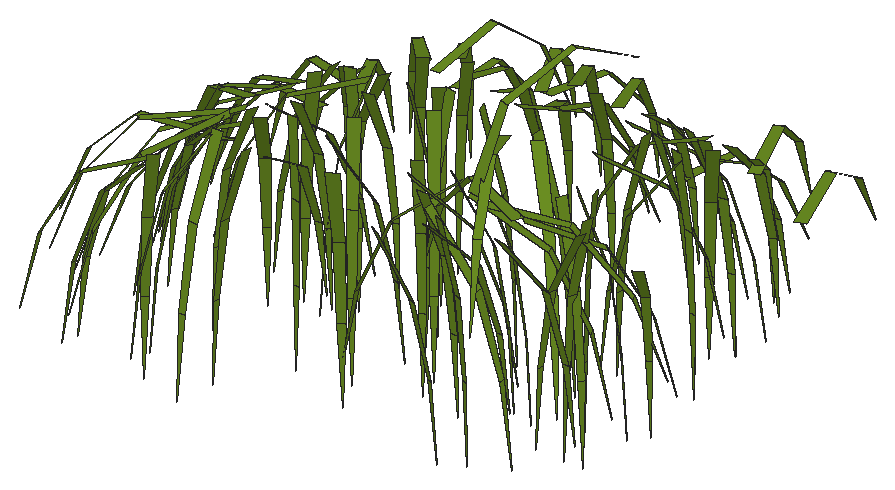
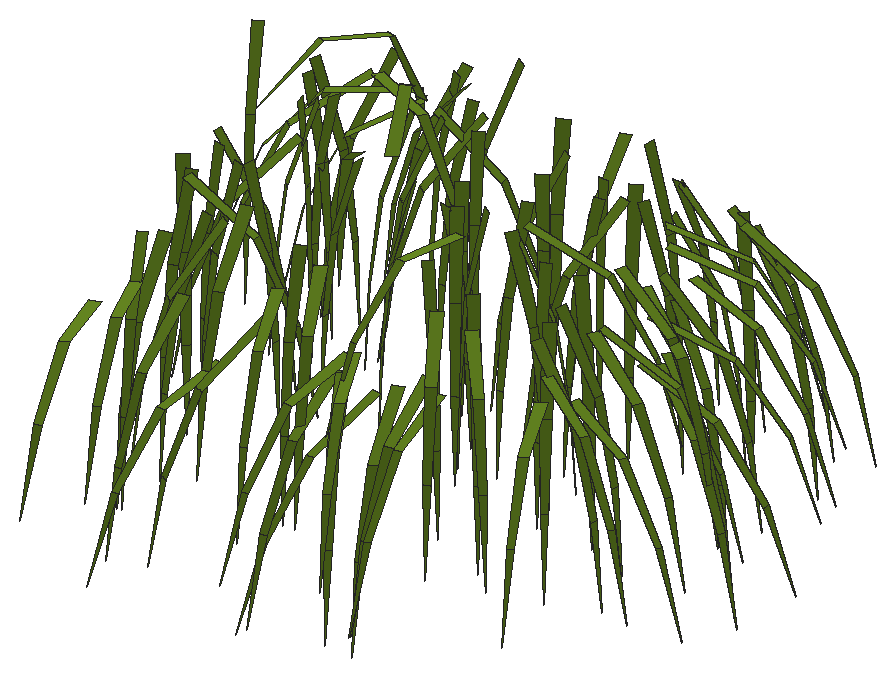
# SketchUp Ruby script. Lengths in inches.
U = 1.inch
M = Sketchup.active_model
def pt(a) = Geom::Point3d.new(a.map { |v| v * U })
def face(e, loops, mat)
  f = e.add_face(loops[0].map { |a| pt(a) })
  loops[1..].each { |l| e.add_face(l.map { |a| pt(a) }).erase! }
  f.material = f.back_material = mat if mat
  f
end
# faces: each face lists its corners as indices into pts; further lists are holes
def faces(e, pts, list, mat = nil) = list.each { |f| face(e, (f[0].is_a?(Array) ? f : [f]).map { |l| l.map { |i| pts[i] } }, mat) }
# xy, xz, yz: faces in a plane at the given z, y or x. An outline is a flat list of corners, or four numbers for a rectangle; further outlines are holes
def ring(l) = l.size == 4 ? [[l[0], l[1]], [l[2], l[1]], [l[2], l[3]], [l[0], l[3]]] : l.each_slice(2).to_a
def flat(e, list, mat, &to3) = list.each { |f| face(e, (f[0].is_a?(Array) ? f : [f]).map { |l| ring(l).map { |u, v| to3.(u, v) } }, mat) }
def xy(e, z, list, mat = nil) = flat(e, list, mat) { |x, y| [x, y, z] }
def xz(e, y, list, mat = nil) = flat(e, list, mat) { |x, z| [x, y, z] }
def yz(e, x, list, mat = nil) = flat(e, list, mat) { |y, z| [x, y, z] }
def lines(e, pts, list) = list.each { |a, b| e.add_line(pt(pts[a]), pt(pts[b])) }
# prism: a flat outline (further loops are holes) pulled along v
def prism(e, loops, v, mat = nil)
  f = face(e, loops, mat); d = Geom::Vector3d.new(v.map { |x| x * U })
  f.pushpull(f.normal.samedirection?(d) ? d.length : -d.length)
end
def box(e, o, s, mat = nil) = prism(e, [[o, [o[0] + s[0], o[1], o[2]], [o[0] + s[0], o[1] + s[1], o[2]], [o[0], o[1] + s[1], o[2]]]], [0, 0, s[2]], mat)
def at(x, y, z, deg = 0) = Geom::Transformation.translation(pt([x, y, z])) * Geom::Transformation.rotation(ORIGIN, Z_AXIS, deg.degrees)
def axes(o, x, y, z) = Geom::Transformation.new([*x, 0, *y, 0, *z, 0, *pt(o).to_a, 1])
def part(name) = M.definitions.add(name)
# library, detail: a bought-in or finely detailed component or shape, given as its bounding box
def library(name, o, s) = part(name).tap { |d| box(d.entities, o, s) }
def detail(e, o, s) = box(e.add_group.entities, o, s)
def put(e, d, t, mat = nil) = e.add_instance(d, t).tap { |i| i.material = mat if mat }
def group(e, t, mat = nil) = e.add_group.tap { |g| g.transformation = t; g.material = mat if mat }.entities
root = M.entities
M.materials.add("[0061_OliveDrab]").color = [107, 142, 35]
p = [[550.11,21.29,553.3],[550.25,21.43,553.3],[550.08,21.45,550.68],[549.24,29.09,553.35],[549.29,29.29,553.35],[548.93,29.29,550.75],
  [559.71,34.42,553.29],[559.91,34.35,553.29],[559.98,34.88,550.71],[553.87,34.64,553.24],[554.06,34.76,553.24],[553.6,35.27,550.71],
  [552.81,34.65,553.26],[553,34.73,553.26],[552.64,35.34,550.73],[547.85,25.41,553.35],[547.93,25.58,553.35],[547.51,25.69,550.77],
  [546.58,26.92,553.23],[546.6875,27.11,553.23],[545.84,27.47,550.77],[546.375,27.2,553.16],[546.48,27.39,553.16],[545.48,27.81,550.77],
  [550.45,29.67,553.38],[550.625,29.79,553.38],[550.4,29.93,550.76],[546.18,25.6,553.38],[546.16,25.82,553.38],[545.23,25.63,550.93],
  [551.1,26.88,553.56],[551.24,27.06,553.56],[551.07,27.04,550.93],[560.84,34.95,553.45],[561.03,34.98,553.45],[560.84,35.57,550.9],
  [555.43,35.47,553.27],[555.62,35.44,553.27],[555.68,36.49,550.86],[549.72,27.6,553.58],[549.75,27.81,553.58],[549.47,27.74,550.97],
  [552.66,27.23,553.71],[552.87,27.28,553.71],[552.75,27.3,551.09],[552.4375,30.0625,553.74],[552.58,30.19,553.74],[552.39,30.26,551.12],
  [562.04,31.48,553.76],[562.24,31.44,553.76],[562.17,31.6,551.14],[555.42,35.49,553.54],[555.625,35.52,553.54],[555.38,36.375,551.07],
  [548.125,21.26,553.77],[548.2,21.46,553.77],[547.77,21.5,551.18],[548.1,23.9,553.91],[548.09,24.12,553.91],[547.6875,23.99,551.3125],
  [561.91,33.37,553.93],[562.13,33.43,553.93],[561.92,33.78,551.33],[559.81,36.35,553.65],[560.01,36.36,553.65],[559.9,37.58,551.33],
  [550.32,21.65,554.01],[550.24,21.84,554.01],[550.11,21.67,551.39],[557.81,31.59,554.03],[557.99,31.69,554.03],[557.8125,31.82,551.41],
  [546.45,29.8,553.84],[546.52,29.98,553.84],[545.39,30.29,551.49],[554.02,29.83,554.14],[554.15,29.97,554.14],[553.97,30.01,551.52],
  [562.45,31.98,554.125],[562.64,31.86,554.125],[562.72,32.2,551.52],[561.72,33.55,554.1],[561.88,33.64,554.1],[561.55,34.03,551.53],
  [552.59,34.7,553.97],[552.8,34.74,553.97],[552.51,35.52,551.47],[552.69,19.91,554.24],[552.5,19.91,554.24],[552.59,19.71,551.62],
  [548.6,20.23,554.24],[548.57,20.43,554.24],[548.2,20.28,551.65],[553.9,23.06,554.21],[554.09,23.04,554.21],[553.99,23.0625,551.59],
  [562.7,24.45,554.26],[562.65,24.64,554.26],[562.65,24.54,551.64],[552.78,25.82,554.18],[552.66,25.99,554.18],[552.59,25.82,551.56],
  [547.35,26.06,554.17],[547.32,26.24,554.17],[546.69,26.04,551.63],[555.71,26.83,554.27],[555.875,26.72,554.27],[555.83,26.83,551.64],
  [563.1875,28.38,554.26],[563.4,28.34,554.26],[563.3,28.41,551.64],[560.79,21.68,554.32],[560.98,21.58,554.32],[560.92,21.69,551.7],
  [556.29,21.94,554.36],[556.5,22.03,554.36],[556.36,22.07,551.74],[551.07,23.2,554.28],[551.125,23.39,554.28],[550.9375,23.33,551.66],
  [555.78,23.36,554.29],[555.6,23.24,554.29],[555.73,23.24,551.67],[562.88,23.37,554.33],[562.91,23.57,554.33],[562.81,23.49,551.71],
  [557.64,23.74,554.33],[557.8125,23.84,554.33],[557.66,23.89,551.71],[557.48,24.76,554.36],[557.3125,24.63,554.36],[557.45,24.625,551.74],
  [556.35,25.86,554.29],[556.15,25.89,554.29],[556.23,25.76,551.66],[558.48,26.8,554.35],[558.55,26.6,554.35],[558.61,26.73,551.72],
  [561.01,27.99,554.27],[561.02,28.22,554.27],[560.92,28.11,551.65],[562.38,29.33,554.29],[562.57,29.28,554.29],[562.51,29.42,551.67],
  [562.67,30.65,554.31],[562.87,30.7,554.31],[562.72,30.89,551.69],[553.05,20.7,554.41],[553.07,20.9,554.41],[552.93,20.8125,551.79],
  [547,23.57,554.32],[546.92,23.77,554.32],[546.21,23.34,551.82],[563.44,23.56,554.4],[563.36,23.39,554.4],[563.49,23.4375,551.77],
  [560.82,24.3125,554.42],[560.97,24.2,554.42],[560.97,24.36,551.79],[563.29,25.32,554.41],[563.45,25.16,554.41],[563.46,25.33,551.79],
  [560.77,26.42,554.39],[560.77,26.2,554.39],[560.9,26.3125,551.77],[562.48,29.92,554.45],[562.65,30.07,554.45],[562.43,30.14,551.83],
  [550.68,20.46,554.49],[550.6,20.64,554.49],[550.43,20.44,551.87],[560.26,20.83,554.53],[560.46,20.72,554.53],[560.47,20.98,551.91],
  [559.15,23.21,554.49],[559.35,23.22,554.49],[559.25,23.38,551.87],[560.18,24.375,554.54],[560.33,24.26,554.54],[560.34,24.43,551.92],
  [552.99,25.53,554.54],[553.18,25.57,554.54],[553.03,25.78,551.93],[552.37,27.28,554.55],[552.46,27.47,554.55],[552.17,27.5,551.94],
  [555.09,27.68,554.48],[555.27,27.81,554.48],[555.08,27.88,551.86],[552.16,35.13,554.3125],[552.34,35.17,554.3125],[552.01,36.23,551.93],
  [562.32,22.95,554.64],[562.37,23.14,554.64],[562.14,23.1,552.02],[554.26,26.83,554.57],[554.44,26.875,554.57],[554.3,27.05,551.96],
  [548.89,33.08,554.34],[549.07,33.18,554.34],[548.38,34.23,552.04],[547.33,20.33,554.66],[547.3125,20.55,554.66],[546.67,20.4,552.11],
  [556.375,24.27,554.71],[556.56,24.17,554.71],[556.59,24.44,552.1],[551.87,24.3,554.72],[552.05,24.42,554.72],[551.77,24.63,552.11],
  [547.21,28.46,554.54],[547.29,28.66,554.54],[546.39,28.91,552.09],[547.35,30.72,554.47],[547.44,30.89,554.47],[546.47,31.29,552.07],
  [562.96,23.25,554.89],[563.18,23.21,554.89],[563.13,23.54,552.28],[561.41,27.05,554.87],[561.4,27.24,554.87],[561.125,27.13,552.26],
  [562.43,21.38,555.01],[562.43,21.2,555.01],[562.78,21.29,552.4],[555.87,35.75,554.78],[556.08,35.74,554.78],[555.99,36.79,552.37],
  [560.8125,23.1,555.15],[561.02,23.07,555.15],[560.96,23.46,552.55],[559.89,24.53,555.1],[560.06,24.42,555.1],[560.18,24.8,552.51],
  [547.37,26.64,555.03],[547.46,26.83,555.03],[546.72,27.08,552.52],[564.9375,24.3,555.21],[565.09,24.4,555.21],[564.8,24.69,552.62],
  [559.88,32.47,555.15],[560.09,32.53,555.15],[559.84,32.97,552.57],[562.52,36.23,554.75],[562.72,36.3,554.75],[562.09,37.7,552.62],
  [547.93,26.11,555.28],[547.99,26.3125,555.28],[547.3,26.4,552.74],[553.48,26.33,555.3125],[553.68,26.29,555.3125],[553.67,26.82,552.74],
  [551.89,32.88,555.18],[552.07,33.01,555.18],[551.5625,33.55,552.66],[549.2,20.37,555.32],[549.06,20.53,555.32],[548.66,20.02,552.78],
  [556.78,22.08,555.42],[556.74,22.28,555.42],[556.29,22.09,552.84],[550.25,32.55,555.29],[550.4,32.68,555.29],[549.66,33.34,552.86],
  [556.77,34.63,555.39],[556.9375,34.72,555.39],[556.44,35.5,552.93],[546.26,23.77,555.38],[546.29,23.96,555.38],[545.13,24.04,553.02],
  [563.03,29.2,555.6],[563.23,29.11,555.6],[563.36,29.61,553.03],[553.4,35.27,555.4],[553.58,35.37,555.4],[552.86,36.43,553.11],
  [562.49,23.64,555.72],[562.33,23.48,555.72],[562.85,23.13,553.17],[563.4,23.97,555.72],[563.49,23.77,555.72],[563.95,24.09,553.15],
  [553.9375,23.94,555.77],[554.13,24,555.77],[553.87,24.53,553.21],[547.92,26.1,555.33],[548.07,26.36,555.33],[547.84,26.37,555.17],
  [547.99,26.64,555.17],[554.55,33.48,555.5],[554.82,33.65,555.5],[555.74,33.52,555.67],[555.93,33.64,555.67],[555.4375,34.25,553.17],
  [550.36,21.02,555.9],[550.54,21.23,555.9],[547.46,21.98,555.77],[547.4,22.17,555.77],[546.58,21.8,553.3],[559.3125,33.39,555.67],
  [559.6,33.29,555.67],[553.29,33.37,555.5],[553.5625,33.48,555.5],[555.14,33.82,555.29],[555.4,33.78,555.29],[560.98,35.61,555.58],
  [561.18,35.7,555.58],[560.5625,36.82,553.29],[548.6875,24.93,555.79],[548.81,25.16,555.79],[547.77,25.7,555.47],[547.74,26,555.47],
  [550.02,28.8125,555.84],[550.1,29.1,555.84],[550.78,29.125,555.93],[551.02,29.3,555.93],[559.27,29.27,555.9],[559.27,29.47,555.9],
  [558.5625,29.38,553.38],[560.99,33.7,555.75],[561.27,33.74,555.75],[550.53,24.83,556.05],[550.47,25.05,556.05],[549.83,24.76,553.52],
  [564.41,25.28,556.01],[564.59,25.15,556.01],[564.875,25.72,553.46],[555.64,33.9375,555.65],[555.92,33.98,555.65],[551.32,26.65,556.16],
  [551.52,26.9,556.16],[550.34,27.47,556.13],[550.38,27.77,556.13],[552.66,27.07,556.33],[552.95,27.14,556.33],[552.74,29.67,556.32],
  [552.94,29.85,556.32],[559.79,34.38,555.38],[560.06,34.38,555.38],[548.98,20.9,556.23],[549.08,21.17,556.23],[548.2,29.11,555.67],
  [548.29,29.36,555.67],[561.93,31.08,556.35],[562.21,31.03,556.35],[549.02,23.89,556.36],[549.01,24.21,556.36],[562.09,32.49,556.39],
  [562.4,32.57,556.39],[550.79,21.8,556.59],[550.68,22.07,556.59],[558.01,31.08,556.59],[558.27,31.21,556.59],[552.89,33.2,556.1],
  [553.1875,33.26,556.1],[554.33,29.49,556.72],[554.51,29.68,556.72],[562,31.39,556.64],[562.27,31.21,556.64],[562.23,32.58,556.49],
  [562.46,32.71,556.49],[552.74,20.36,556.82],[552.47,20.37,556.82],[549.49,20.3,556.71],[549.45,20.59,556.71],[553.85,23.03,556.84],
  [554.125,23,556.84],[553.12,26,556.77],[552.96,26.24,556.77],[548.64,26.24,556.45],[548.6,26.5,556.45],[560.66,21.51,556.94],
  [560.9375,21.38,556.94],[551.49,23.04,556.86],[551.5625,23.32,556.86],[555.72,23.53,556.91],[555.47,23.36,556.91],[563.1,23.29,556.95],
  [563.15,23.58,556.95],[557.73,23.49,556.94],[557.98,23.625,556.94],[548.4,24.13,556.47],[548.27,24.41,556.47],[562.79,24.43,556.88],
  [562.71,24.7,556.88],[556.42,26.11,556.9],[556.14,26.15,556.9],[555.57,26.69,556.88],[555.8,26.53,556.88],[558.23,26.76,556.96],
  [558.32,26.47,556.96],[561.27,27.9375,556.89],[561.28,28.25,556.89],[563.12,28.25,556.88],[563.41,28.19,556.88],[562.26,29.03,556.89],
  [562.53,28.96,556.89],[562.74,30.14,556.88],[563.02,30.2,556.88],[549.8,31.3,556.05],[550.0625,31.44,556.05],[552.53,33.31,556.17],
  [552.78,33.37,556.17],[553.37,20.61,557.01],[553.41,20.9,557.01],[556.35,21.6875,556.98],[556.65,21.82,556.98],[563.18,23.71,557],
  [563.08,23.47,557],[560.59,24.07,557.02],[560.8,23.91,557.02],[557.35,24.99,556.98],[557.12,24.8,556.98],[563.02,25.13,557.02],
  [563.24,24.9,557.02],[560.45,26.46,557],[560.46,26.14,557],[562.79,29.52,557.02],[563.02,29.73,557.02],[559.98,20.4,557.1],
  [560.25,20.25,557.1],[551.25,20.68,557.04],[551.13,20.93,557.04],[559.13,22.8,557.08],[559.41,22.81,557.08],[559.91,24.07,557.14],
  [560.125,23.91,557.14],[553.08,24.97,557.11],[553.34,25.03,557.11],[555.32,27.3,557.07],[555.5625,27.48,557.07],[548.68,27.83,556.62],
  [548.8,28.11,556.62],[548.92,29.85,556.4],[549.04,30.09,556.4],[562.82,22.78,557.21],[562.89,23.04,557.21],[554.34,26.33,557.15],
  [554.6,26.39,557.15],[552.92,26.96,557.1],[553.05,27.23,557.1],[548.64,20.38,556.93],[548.62,20.68,556.93],[556.06,23.76,557.27],
  [556.32,23.625,557.27],[552.24,23.67,557.24],[552.49,23.84,557.24],[564.71,24.13,557.18],[564.79,23.95,557.18],[565.23,24.21,555.85],
  [565.59,24.42,554.72],[563.26,34.11,556.11],[563.54,34.21,556.11],[555.8,33.9375,556.68],[556.09,33.93,556.68],[562.78,22.55,557.41],
  [563.08,22.49,557.41],[562.1,27.05,557.4],[562.08,27.32,557.4],[561.63,21.42,557.51],[561.63,21.16,557.51],[548.68,25.93,557.1875],
  [548.82,26.21,557.1875],[560.67,22.25,557.63],[560.97,22.21,557.63],[559.38,23.83,557.58],[559.63,23.67,557.58],[560.15,31.42,557.54],
  [560.45,31.51,557.54],[565.39,23.52,557.67],[565.61,23.66,557.67],[549.93,25.21,556.26],[550.11,25.54,556.26],[552.67,31.67,557.375],
  [552.93,31.85,557.375],[550.19,21.21,557.6],[549.99,21.4375,557.6],[558.08,23.97,557.69],[558.17,24.15,557.69],[557.19,24.48,555.27],
  [549.97,24.89,556.44],[550.15,25.2,556.44],[553.23,25.26,557.7],[553.52,25.21,557.7],[549.25,25.68,557.51],[549.33,25.97,557.51],
  [551.38,31.26,557.28],[551.59,31.46,557.28],[554.74,31.45,556.35],[555.06,31.4,556.35],[557.8,22.25,557.83],[557.74,22.53,557.83],
  [548.12,23.45,557.21],[548.16,23.71,557.21],[559.78,31.77,555.64],[560.12,31.77,555.64],[557.48,33.09,557.39],[557.72,33.21,557.39],
  [554.37,33.47,557.05],[554.62,33.62,557.05],[550.16,25.875,556.54],[550.125,26.25,556.54],[554.15,31.17,556.65],[554.49,31.3125,556.65],
  [555.78,31.46,556.64],[556.11,31.67,556.64],[562.5,28.24,557.99],[562.78,28.11,557.99],[561.78,33.71,557.2],[562.0625,33.83,557.2],
  [562.32,23.55,558.07],[562.44,23.27,558.07],[561.64,24.52,558.05],[561.43,24.3,558.05],[550.6,28.19,556.21],[550.71,28.5,556.21],
  [558.59,31.39,557.2],[558.9375,31.27,557.2],[556,31.54,556.65],[556.35,31.59,556.65],[555.09,32.09,558.04],[555.28,32.09,558.04],
  [555.24,32.5625,557.11],[555.17,33.28,555.7],[556.47,32.2,557.82],[556.74,32.35,557.82],[549.03,22.44,557.82],[548.94,22.72,557.82],
  [554.23,22.78,558.11],[554.5,22.86,558.11],[550.46,23.98,557.49],[550.6,24.26,557.49],[551.78,28.26,557.71],[551.88,28.61,557.71],
  [561.3125,31.42,557.02],[561.65,31.48,557.02],[551.05,20.37,558.35],[551.28,20.63,558.35],[551.67,27.8,558.01],[551.97,28.02,558.01],
  [560.67,29.2,558.12],[560.68,29.48,558.12],[564.15,31.64,555.95],[564.49,31.77,555.95],[563.61,24.27,558.29],[563.86,24.08,558.29],
  [551.02,28.99,556.31],[551.33,29.16,556.31],[551.875,25.15,558.28],[551.79,25.46,558.28],[551.8,27.24,558.3],[551.85,27.61,558.3],
  [553.41,30.8,557.03],[553.77,30.88,557.03],[550.8,20.18,557.98],[550.92,20.52,557.98],[551.93,26.13,558.66],[552.17,26.43,558.66],
  [553.0625,30.78,556.59],[553.37,30.85,556.59],[552.73,26.65,558.92],[553.08,26.73,558.92],[553.6,28.66,558.58],[553.85,28.88,558.58],
  [550.97,23.95,558.125],[550.95,24.33,558.125],[550.96,26.61,557.625],[550.91,26.92,557.625],[551.17,28.625,556.98],[551.32,28.92,556.98],
  [561.71,29.97,558.72],[562.05,29.91,558.72],[562.53,30.62,558.18],[562.91,30.72,558.18],[550.62,25.0625,557.51],[550.47,25.41,557.51],
  [563.29,30.71,558],[563.5625,30.87,558],[552.01,22.28,558.87],[551.87,22.6,558.87],[550.92,26.89,557.625],[551.0625,27.24,557.625],
  [558.62,29.77,558.79],[558.94,29.93,558.79],[561.09,30.0625,558.72],[561.42,29.85,558.72],[561.58,21.49,558.96],[561.39,21.375,558.96],
  [562.17,20.25,556.72],[551.4,20.52,558.49],[551.36,20.875,558.49],[555.21,28.6,559.03],[555.43,28.84,559.03],[555.73,31.35,557.11],
  [556.09,31.34,557.11],[552.78,21.42,559.22],[552.45,21.42,559.22],[553.8125,22.93,559.46],[554.15,22.9,559.46],[553.93,26.5,559.22],
  [553.73,26.8,559.22],[550.97,20.5,558.13],[550.95,20.87,558.13],[560.39,21.01,559.5],[560.73,20.85,559.5],[552.59,22.72,559.23],
  [552.68,23.06,559.23],[557.99,22.96,559.5],[558.29,23.13,559.5],[563.69,23.17,559.5],[563.75,23.52,559.5],[555.52,23.91,559.5],
  [555.21,23.71,559.5],[563,24.46,559.5],[562.9,24.79,559.5],[555.22,26.23,559.44],[555.52,26.04,559.44],[556.53,26.65,559.46],
  [556.18,26.7,559.46],[563.01,27.84,559.47],[563.37,27.77,559.47],[561.95,27.875,559.42],[561.97,28.26,559.42],[562.02,28.26,559.39],
  [562.36,28.17,559.39],[562.97,28.99,559.23],[563.32,29.07,559.23],[554.1875,20.47,559.5],[554.23,20.82,559.5],[552.6,21.29,559.21],
  [552.45,21.6,559.21],[556.61,21.02,559.5],[556.97,21.18,559.5],[560.05,23.41,559.5],[560.31,23.21,559.5],[562.45,24.06,559.5],
  [562.32,23.76,559.5],[562.39,24.57,559.5],[562.66,24.29,559.5],[556.93,25.57,559.5],[556.64,25.34,559.5],[559.66,26.47,559.5],
  [559.67,26.09,559.5],[557.6,26.57,559.5],[557.72,26.23,559.5],[563.63,28.53,559.3],[563.91,28.78,559.3],[559.43,19.48,559.5],
  [559.77,19.3,559.5],[559.14,21.79,559.5],[559.48,21.8,559.5],[559.2,23.17,559.5],[559.47,22.98,559.5],[553.34,23.65,559.36],
  [553.67,23.72,559.36],[554.61,25.1,559.45],[554.93,25.18,559.45],[554.2,26.29,559.29],[554.36,26.62,559.29],[555.9375,26.41,559.46],
  [556.23,26.64,559.46],[555.64,31.18,557.18],[555.94,31.35,557.18],[562.82,31.3,557.13],[563.16,31.45,557.13],[553.08,22.36,559.35],
  [553.39,22.57,559.35],[564.05,22.42,559.5],[564.14,22.74,559.5],[550.66,23.03,557.71],[550.71,23.35,557.71],[563.12,23.46,559.16],
  [563.23,23.21,559.16],[550.86,24.79,558.09],[551.04,25.13,558.09],[555.38,22.57,559.5],[555.7,22.4,559.5],[553.07,29.38,557.99],
  [553.33,29.62,557.99],[562.43,21.01,559.5],[562.8,20.93,559.5],[563.68,27.11,559.5],[563.66,27.43,559.5],[554.04,29.64,558.32],
  [554.36,29.86,558.32],[558.59,30.77,557.92],[558.89,30.92,557.92],[559.93,21.45,559.5],[559.93,21.13,559.5],[551.56,24.98,558.54],
  [551.66,25.33,558.54],[560.74,29.37,559.07],[561.11,29.48,559.07],[560.42,20.43,559.5],[560.79,20.38,559.5],[551.95,22.76,558.79],
  [551.69,23.04,558.79],[558.38,22.35,559.5],[558.6875,22.15,559.5],[566.38,21.91,559.5],[566.65,22.09,559.5],[552.82,23.21,559.29],
  [553.17,23.15,559.29],[559.78,23.17,559.52],[559.9,23.43,559.52],[559.79,22.63,559.5],[559.72,22.98,559.5],[551.45,23.19,558.51],
  [551.34,23.53,558.51],[557.71,30.02,558.61],[558.04,30.22,558.61],[560.1,26.0625,559.5],[559.83,25.79,559.5],[561.51,26.34,559.5],
  [561.85,26.17,559.5],[555.08,30.03,559.66],[555.34,30.03,559.66],[554.8125,20.63,559.5],[555.14,20.73,559.5],[560.28,22.72,559.5],
  [560.34,22.58,559.5],[560.43,22.37,559.5],[563.08,29.12,559.16],[563.09,29.47,559.16],[562.2,22.41,559.5],[562.29,22.35,559.5],
  [562.51,22.18,559.5],[554.21,25.75,559.32],[554.11,26.125,559.32],[560.49,23.45,560.3125],[560.22,23.3,560.3125],[560.93,22.14,559.49],
  [560.73,22.43,559.5],[560.875,22.11,559.5],[555.08,27.43,559.29],[555.4,27.43,559.29],[562.16,22.08,559.5],[562.31,22.4,559.5],
  [560.28,22.59,559.5],[560.65,22.53,559.5],[560.79,23.62,561.88],[560.49,23.67,561.88],[559.26,25.63,559.5],[558.93,25.4375,559.5],
  [560.93,26.14,562.65],[561.14,26.1,562.65],[561.41,28.43,561.45]]
faces(root,p,[[0,1,2],[3,4,5],[6,7,8],[9,10,11],[12,13,14],[15,16,17],[18,19,20],[21,22,23],
  [24,25,26],[27,28,29],[30,31,32],[33,34,35],[36,37,38],[39,40,41],[42,43,44],[45,46,47],
  [48,49,50],[51,52,53],[54,55,56],[57,58,59],[60,61,62],[63,64,65],[66,67,68],[69,70,71],
  [72,73,74],[75,76,77],[78,79,80],[81,82,83],[84,85,86],[87,88,89],[90,91,92],[93,94,95],
  [96,97,98],[99,100,101],[102,103,104],[105,106,107],[108,109,110],[111,112,113],[114,115,116],[117,118,119],
  [120,121,122],[123,124,125],[126,127,128],[129,130,131],[132,133,134],[135,136,137],[138,139,140],[141,142,143],
  [144,145,146],[147,148,149],[150,151,152],[153,154,155],[156,157,158],[159,160,161],[162,163,164],[165,166,167],
  [168,169,170],[171,172,173],[174,175,176],[177,178,179],[180,181,182],[183,184,185],[186,187,188],[189,190,191],
  [192,193,194],[195,196,197],[198,199,200],[201,202,203],[204,205,206],[207,208,209],[210,211,212],[213,214,215],
  [216,217,218],[219,220,221],[222,223,224],[225,226,227],[228,229,230],[231,232,233],[234,235,236],[237,238,239],
  [240,241,242],[243,244,245],[246,247,248],[249,250,251],[252,253,254],[255,256,257],[258,259,260],[261,262,263],
  [264,265,266],[267,268,269],[270,271,272],[273,274,275],[276,277,278],[279,280,281],[282,283,284],[285,286,19,18],
  [287,288,22,21],[289,290,10,9],[291,292,293],[294,295,1,0],[296,297,298],[299,300,7,6],[301,302,13,12],[303,304,37,36],
  [305,306,307],[308,309,16,15],[310,311,28,27],[312,313,4,3],[314,315,25,24],[316,317,318],[319,320,34,33],[321,322,323],
  [324,325,326],[327,328,52,51],[329,330,31,30],[331,332,40,39],[333,334,43,42],[335,336,46,45],[337,338,64,63],[339,340,55,54],
  [341,342,73,72],[343,344,49,48],[345,346,58,57],[347,348,61,60],[349,350,67,66],[351,352,70,69],[353,354,85,84],[355,356,76,75],
  [357,358,79,78],[359,360,82,81],[361,362,88,87],[363,364,91,90],[365,366,94,93],[367,368,100,99],[369,370,103,102],[371,372,112,111],
  [373,374,118,117],[375,376,121,120],[377,378,124,123],[379,380,127,126],[381,382,151,150],[383,384,97,96],[385,386,133,132],[387,388,106,105],
  [389,390,136,135],[391,392,139,138],[393,394,109,108],[395,396,142,141],[397,398,145,144],[399,400,199,198],[401,402,190,189],[403,404,148,147],
  [405,406,115,114],[407,408,154,153],[409,410,157,156],[411,412,130,129],[413,414,160,159],[415,416,163,162],[417,418,166,165],[419,420,172,171],
  [421,422,169,168],[423,424,175,174],[425,426,178,177],[427,428,181,180],[429,430,187,186],[431,432,211,210],[433,434,214,213],[435,436,193,192],
  [437,438,196,195],[439,440,184,183],[441,442,202,201],[443,444,205,204],[445,446,208,207],[447,448,449,450],[451,452,244,243],[453,454,226,225],
  [455,456,217,216],[457,458,220,219],[459,460,223,222],[461,462,235,234],[463,464,229,228],[465,466,232,231],[467,468,241,240],[469,470,449,238,237],
  [471,472,288,287],[473,474,253,252],[475,476,256,255],[477,478,479],[480,481,286,285],[482,483,250,249],[484,485,247,246],[486,487,262,261],
  [488,489,304,303],[490,491,259,258],[492,493,268,267],[494,495,338,337],[496,497,265,264],[498,499,274,273],[500,501,311,310],[502,503,302,301],
  [504,505,290,289],[506,507,271,270],[508,509,306,305],[510,511,280,279],[512,513,277,276],[514,515,342,341],[516,517,300,299],[518,519,328,327],
  [520,521,522,523],[524,525,292,291],[526,527,297,296],[528,529,283,282],[530,531,309,308],[532,533,313,312],[534,535,320,319],[536,537,295,294],
  [538,539,315,314],[540,541,317,316],[542,543,452,451],[544,545,325,324],[546,547,400,399],[548,549,322,321],[550,551,332,331],[552,553,354,353],
  [554,555,340,339],[556,557,330,329],[558,559,402,401],[560,561,334,333],[562,563,336,335],[564,565,346,345],[566,567,370,369],[568,569,434,433],
  [570,571,344,343],[572,573,348,347],[574,575,382,381],[576,577,360,359],[578,579,350,349],[580,581,432,431],[582,583,352,351],[584,585,358,357],
  [586,587,588],[589,590,364,363],[591,592,356,355],[593,594,454,453],[595,596,362,361],[597,598,366,365],[599,600,368,367],[601,602,442,441],
  [603,604,372,371],[605,606,374,373],[607,608,380,379],[609,610,378,377],[611,612,376,375],[613,614,384,383],[615,616,388,387],[617,618,386,385],
  [619,620,394,393],[621,622,392,391],[623,624,396,395],[625,626,398,397],[627,628,404,403],[629,630,422,421],[631,632,406,405],[633,634,410,409],
  [635,636,408,407],[637,638,414,413],[639,640,412,411],[641,642,416,415],[643,644,390,389],[645,646,418,417],[647,648,420,419],[649,650,424,423],
  [651,652,426,425],[653,654,428,427],[655,656,438,437],[657,658,440,439],[659,660,430,429],[661,662,522,499,498],[663,664,509,508],[665,666,446,445],
  [667,668,436,435],[669,670,493,492],[671,672,448,447],[673,674,462,461],[675,676,444,443],[677,678,487,486],[679,680,456,455],[681,682,458,457],
  [683,684,474,473],[685,686,497,496],[687,688,460,459],[689,690,485,484],[691,692,468,467],[693,694,464,463],[695,696,476,475],[697,698,466,465],
  [699,700,470,469],[701,702,483,482],[703,704,478,477],[705,706,491,490],[707,708,527,526],[709,710,525,524],[711,712,513,512],[713,714,507,506],
  [715,716,521,520],[717,718,529,528],[719,720,721,511,510],[722,723,541,540],[724,725,726,545,544],[727,728,549,548],[729,730,731,587,586],[732,733,731,672,671],
  [734,735,716,715],[736,725,737,704,703],[738,720,739,740,741],[742,743,730,729],[744,745,746],[741,740,745,744]],"[0061_OliveDrab]")
